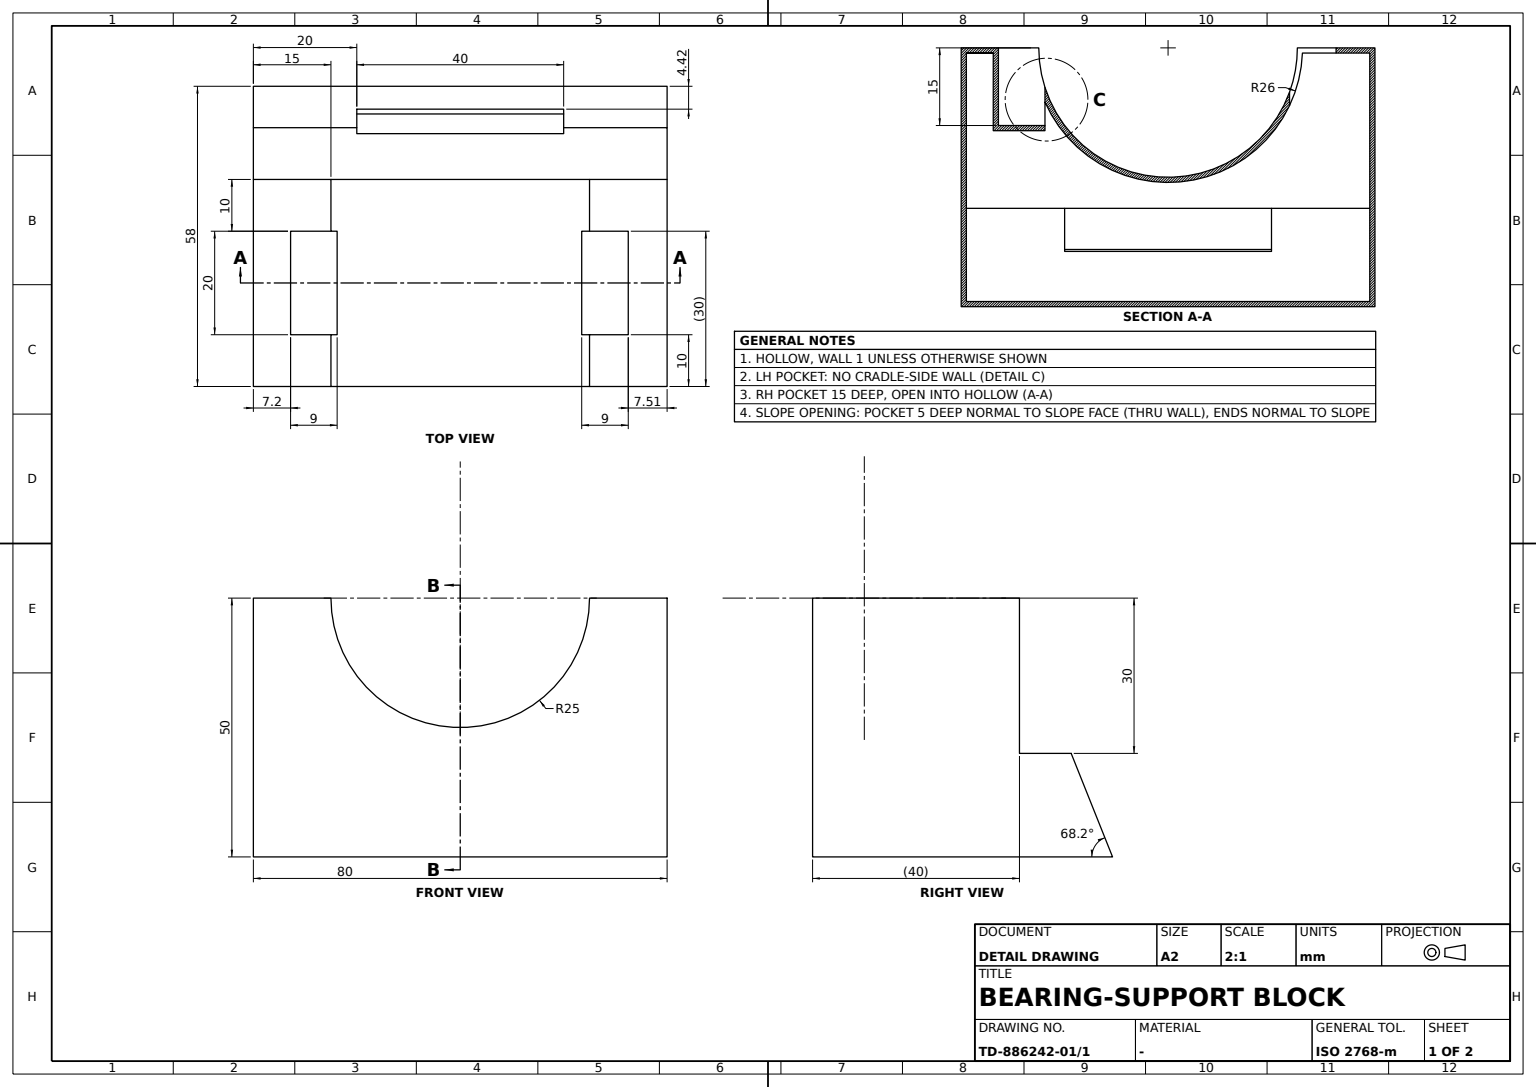
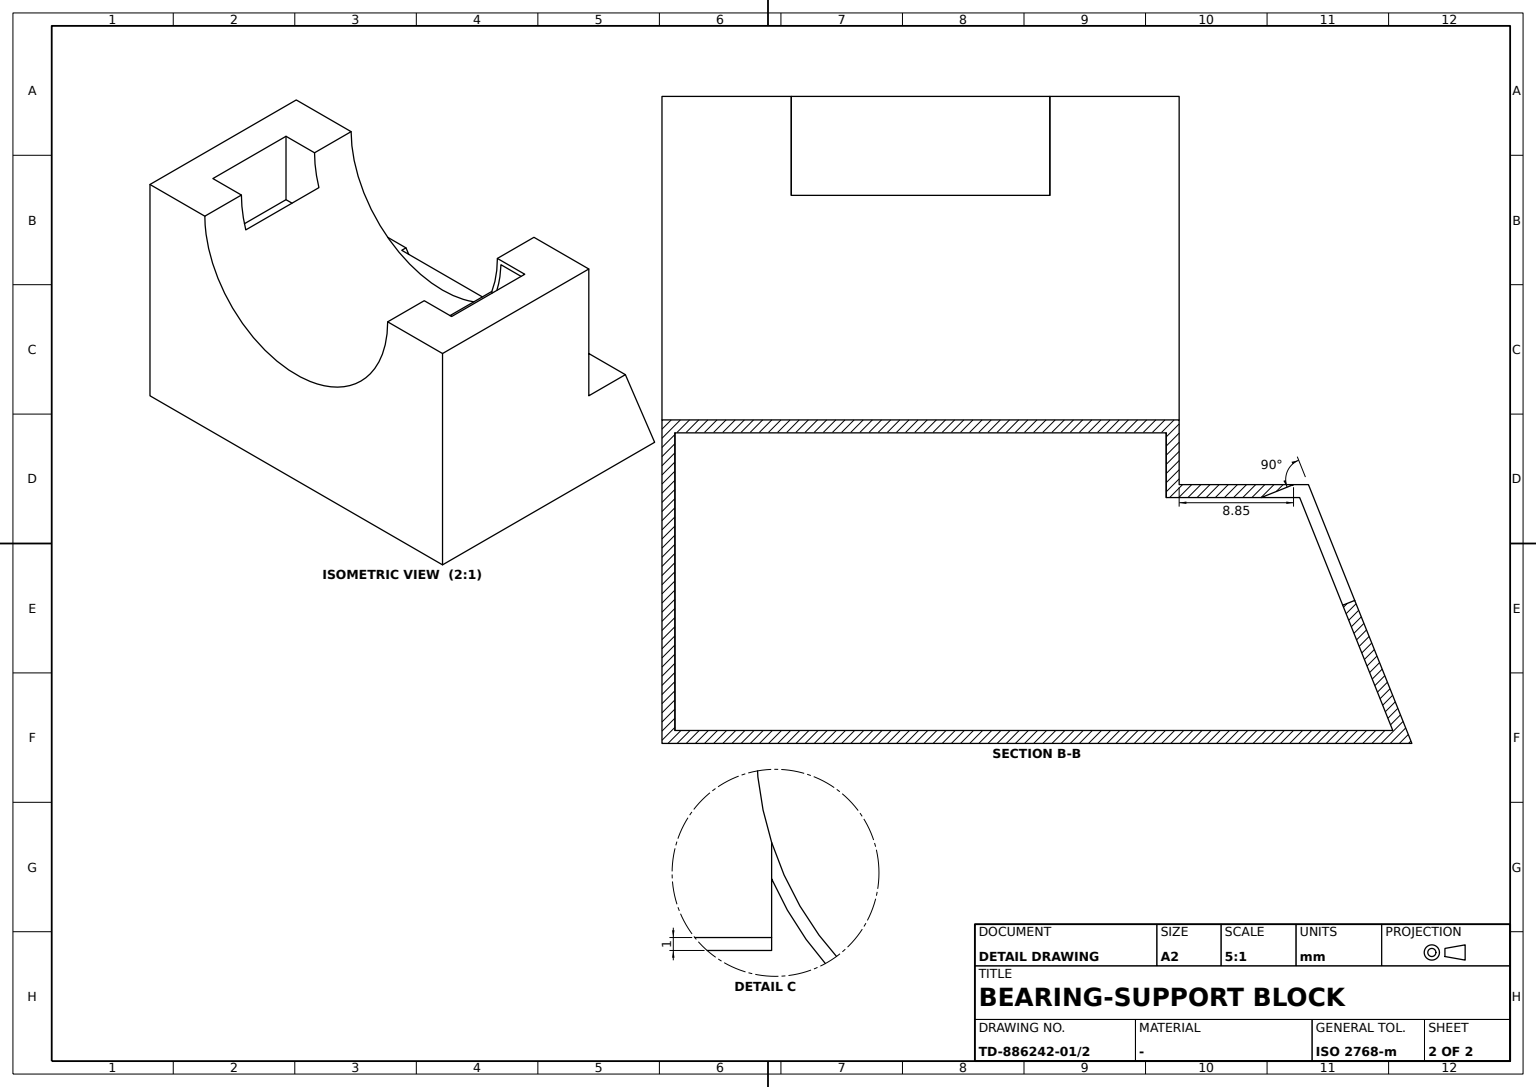
ISO-10303-21;
HEADER;
FILE_DESCRIPTION((''),'2;1');
FILE_NAME('','',(''),(''),'','','');
FILE_SCHEMA(('AUTOMOTIVE_DESIGN'));
ENDSEC;
DATA;
#1=APPLICATION_CONTEXT('');
#2=PRODUCT_CONTEXT('',#1,'mechanical');
#3=PRODUCT('','','',(#2));
#4=PRODUCT_DEFINITION_FORMATION('','',#3);
#5=PRODUCT_DEFINITION_CONTEXT('',#1,'design');
#6=PRODUCT_DEFINITION('','',#4,#5);
#7=PRODUCT_DEFINITION_SHAPE('','',#6);
#8=(LENGTH_UNIT()NAMED_UNIT(*)SI_UNIT(.MILLI.,.METRE.));
#9=(NAMED_UNIT(*)PLANE_ANGLE_UNIT()SI_UNIT($,.RADIAN.));
#10=(NAMED_UNIT(*)SI_UNIT($,.STERADIAN.)SOLID_ANGLE_UNIT());
#11=UNCERTAINTY_MEASURE_WITH_UNIT(LENGTH_MEASURE(0.005),#8,'distance_accuracy_value','');
#12=(GEOMETRIC_REPRESENTATION_CONTEXT(3)GLOBAL_UNCERTAINTY_ASSIGNED_CONTEXT((#11))GLOBAL_UNIT_ASSIGNED_CONTEXT((#8,#9,#10))REPRESENTATION_CONTEXT('',''));
#13=CARTESIAN_POINT('',(-80.,11.,25.));
#14=VERTEX_POINT('',#13);
#15=CARTESIAN_POINT('',(-80.,-29.,25.));
#16=VERTEX_POINT('',#15);
#17=DIRECTION('',(0.,-1.,0.));
#18=VECTOR('',#17,1000.);
#19=LINE('',#13,#18);
#20=EDGE_CURVE('',#14,#16,#19,.T.);
#21=ORIENTED_EDGE('',*,*,#20,.F.);
#22=CARTESIAN_POINT('',(-80.,11.,-5.));
#23=VERTEX_POINT('',#22);
#24=DIRECTION('',(0.,0.,1.));
#25=VECTOR('',#24,1000.);
#26=LINE('',#22,#25);
#27=EDGE_CURVE('',#23,#14,#26,.T.);
#28=ORIENTED_EDGE('',*,*,#27,.F.);
#29=CARTESIAN_POINT('',(-80.,21.,-5.));
#30=VERTEX_POINT('',#29);
#31=LINE('',#29,#18);
#32=EDGE_CURVE('',#30,#23,#31,.T.);
#33=ORIENTED_EDGE('',*,*,#32,.F.);
#34=CARTESIAN_POINT('',(-80.,29.,-25.));
#35=VERTEX_POINT('',#34);
#36=DIRECTION('',(0.,-0.371390676,0.928476691));
#37=VECTOR('',#36,1000.);
#38=LINE('',#34,#37);
#39=EDGE_CURVE('',#35,#30,#38,.T.);
#40=ORIENTED_EDGE('',*,*,#39,.F.);
#41=CARTESIAN_POINT('',(-80.,-29.,-25.));
#42=VERTEX_POINT('',#41);
#43=DIRECTION('',(0.,1.,0.));
#44=VECTOR('',#43,1000.);
#45=LINE('',#41,#44);
#46=EDGE_CURVE('',#42,#35,#45,.T.);
#47=ORIENTED_EDGE('',*,*,#46,.F.);
#48=DIRECTION('',(0.,0.,-1.));
#49=VECTOR('',#48,1000.);
#50=LINE('',#15,#49);
#51=EDGE_CURVE('',#16,#42,#50,.T.);
#52=ORIENTED_EDGE('',*,*,#51,.F.);
#53=EDGE_LOOP('',(#21,#28,#33,#40,#47,#52));
#54=FACE_BOUND('',#53,.T.);
#55=CARTESIAN_POINT('',(-80.,0.,0.));
#56=DIRECTION('',(1.,0.,0.));
#57=AXIS2_PLACEMENT_3D('',#55,#56,#43);
#58=PLANE('',#57);
#59=ADVANCED_FACE('',(#54),#58,.F.);
#60=CARTESIAN_POINT('',(-63.80175,2.,9.));
#61=VERTEX_POINT('',#60);
#62=CARTESIAN_POINT('',(-63.80175,-20.,9.));
#63=VERTEX_POINT('',#62);
#64=CARTESIAN_POINT('',(-63.80175,0.,9.));
#65=LINE('',#64,#18);
#66=EDGE_CURVE('',#61,#63,#65,.T.);
#67=ORIENTED_EDGE('',*,*,#66,.F.);
#68=CARTESIAN_POINT('',(-63.80175,2.,14.536889));
#69=VERTEX_POINT('',#68);
#70=CARTESIAN_POINT('',(-63.80175,2.,25.));
#71=LINE('',#70,#49);
#72=EDGE_CURVE('',#69,#61,#71,.T.);
#73=ORIENTED_EDGE('',*,*,#72,.F.);
#74=CARTESIAN_POINT('',(-63.80175,1.,14.536889));
#75=VERTEX_POINT('',#74);
#76=LINE('',#68,#44);
#77=EDGE_CURVE('',#69,#75,#76,.F.);
#78=ORIENTED_EDGE('',*,*,#77,.T.);
#79=CARTESIAN_POINT('',(-63.80175,1.,10.));
#80=VERTEX_POINT('',#79);
#81=CARTESIAN_POINT('',(-63.80175,1.,25.));
#82=LINE('',#81,#49);
#83=EDGE_CURVE('',#75,#80,#82,.T.);
#84=ORIENTED_EDGE('',*,*,#83,.T.);
#85=CARTESIAN_POINT('',(-63.80175,-19.,10.));
#86=VERTEX_POINT('',#85);
#87=LINE('',#85,#44);
#88=EDGE_CURVE('',#86,#80,#87,.T.);
#89=ORIENTED_EDGE('',*,*,#88,.F.);
#90=CARTESIAN_POINT('',(-63.80175,-19.,14.536889));
#91=VERTEX_POINT('',#90);
#92=CARTESIAN_POINT('',(-63.80175,-19.,25.));
#93=LINE('',#92,#49);
#94=EDGE_CURVE('',#91,#86,#93,.T.);
#95=ORIENTED_EDGE('',*,*,#94,.F.);
#96=CARTESIAN_POINT('',(-63.80175,-20.,14.536889));
#97=VERTEX_POINT('',#96);
#98=LINE('',#90,#44);
#99=EDGE_CURVE('',#91,#97,#98,.F.);
#100=ORIENTED_EDGE('',*,*,#99,.T.);
#101=CARTESIAN_POINT('',(-63.80175,-20.,25.));
#102=LINE('',#101,#49);
#103=EDGE_CURVE('',#97,#63,#102,.T.);
#104=ORIENTED_EDGE('',*,*,#103,.T.);
#105=EDGE_LOOP('',(#67,#73,#78,#84,#89,#95,#100,#104));
#106=FACE_BOUND('',#105,.T.);
#107=DIRECTION('',(-1.,0.,0.));
#108=AXIS2_PLACEMENT_3D('',#92,#107,#43);
#109=PLANE('',#108);
#110=ADVANCED_FACE('',(#106),#109,.F.);
#111=CARTESIAN_POINT('',(-16.511753,-19.,16.438326));
#112=VERTEX_POINT('',#111);
#113=CARTESIAN_POINT('',(-16.511753,-19.,13.850908));
#114=VERTEX_POINT('',#113);
#115=CARTESIAN_POINT('',(-16.511753,-19.,25.));
#116=LINE('',#115,#49);
#117=EDGE_CURVE('',#112,#114,#116,.T.);
#118=ORIENTED_EDGE('',*,*,#117,.F.);
#119=CARTESIAN_POINT('',(-15.,-19.,25.));
#120=VERTEX_POINT('',#119);
#121=CARTESIAN_POINT('',(-40.,-19.,25.));
#122=AXIS2_PLACEMENT_3D('',#121,#17,#48);
#123=CIRCLE('',#122,25.);
#124=EDGE_CURVE('',#112,#120,#123,.T.);
#125=ORIENTED_EDGE('',*,*,#124,.T.);
#126=CARTESIAN_POINT('',(-7.511753,-19.,25.));
#127=VERTEX_POINT('',#126);
#128=CARTESIAN_POINT('',(0.,-19.,25.));
#129=VECTOR('',#107,1000.);
#130=LINE('',#128,#129);
#131=EDGE_CURVE('',#127,#120,#130,.T.);
#132=ORIENTED_EDGE('',*,*,#131,.F.);
#133=CARTESIAN_POINT('',(-7.511753,-19.,24.));
#134=VERTEX_POINT('',#133);
#135=LINE('',#126,#49);
#136=EDGE_CURVE('',#127,#134,#135,.T.);
#137=ORIENTED_EDGE('',*,*,#136,.T.);
#138=CARTESIAN_POINT('',(-14.019238,-19.,24.));
#139=VERTEX_POINT('',#138);
#140=CARTESIAN_POINT('',(-63.80175,-19.,24.));
#141=VECTOR('',#56,1000.);
#142=LINE('',#140,#141);
#143=EDGE_CURVE('',#139,#134,#142,.T.);
#144=ORIENTED_EDGE('',*,*,#143,.F.);
#145=CIRCLE('',#122,26.);
#146=EDGE_CURVE('',#114,#139,#145,.T.);
#147=ORIENTED_EDGE('',*,*,#146,.F.);
#148=EDGE_LOOP('',(#118,#125,#132,#137,#144,#147));
#149=FACE_BOUND('',#148,.T.);
#150=AXIS2_PLACEMENT_3D('',#92,#17,#107);
#151=PLANE('',#150);
#152=ADVANCED_FACE('',(#149),#151,.F.);
#153=ORIENTED_EDGE('',*,*,#27,.T.);
#154=CARTESIAN_POINT('',(-65.,11.,25.));
#155=VERTEX_POINT('',#154);
#156=CARTESIAN_POINT('',(0.,11.,25.));
#157=LINE('',#156,#129);
#158=EDGE_CURVE('',#155,#14,#157,.T.);
#159=ORIENTED_EDGE('',*,*,#158,.F.);
#160=CARTESIAN_POINT('',(-15.,11.,25.));
#161=VERTEX_POINT('',#160);
#162=CARTESIAN_POINT('',(-40.,11.,25.));
#163=AXIS2_PLACEMENT_3D('',#162,#17,#48);
#164=CIRCLE('',#163,25.);
#165=EDGE_CURVE('',#161,#155,#164,.F.);
#166=ORIENTED_EDGE('',*,*,#165,.F.);
#167=VERTEX_POINT('',#156);
#168=EDGE_CURVE('',#167,#161,#157,.T.);
#169=ORIENTED_EDGE('',*,*,#168,.F.);
#170=CARTESIAN_POINT('',(0.,11.,-5.));
#171=VERTEX_POINT('',#170);
#172=LINE('',#170,#25);
#173=EDGE_CURVE('',#171,#167,#172,.T.);
#174=ORIENTED_EDGE('',*,*,#173,.F.);
#175=LINE('',#170,#129);
#176=EDGE_CURVE('',#171,#23,#175,.T.);
#177=ORIENTED_EDGE('',*,*,#176,.T.);
#178=EDGE_LOOP('',(#153,#159,#166,#169,#174,#177));
#179=FACE_BOUND('',#178,.T.);
#180=AXIS2_PLACEMENT_3D('',#170,#17,#24);
#181=PLANE('',#180);
#182=ADVANCED_FACE('',(#179),#181,.F.);
#183=CARTESIAN_POINT('',(0.,29.,-25.));
#184=VERTEX_POINT('',#183);
#185=CARTESIAN_POINT('',(0.,21.,-5.));
#186=VERTEX_POINT('',#185);
#187=LINE('',#183,#37);
#188=EDGE_CURVE('',#184,#186,#187,.T.);
#189=ORIENTED_EDGE('',*,*,#188,.T.);
#190=LINE('',#185,#18);
#191=EDGE_CURVE('',#186,#171,#190,.T.);
#192=ORIENTED_EDGE('',*,*,#191,.T.);
#193=ORIENTED_EDGE('',*,*,#173,.T.);
#194=CARTESIAN_POINT('',(0.,-29.,25.));
#195=VERTEX_POINT('',#194);
#196=LINE('',#156,#18);
#197=EDGE_CURVE('',#167,#195,#196,.T.);
#198=ORIENTED_EDGE('',*,*,#197,.T.);
#199=CARTESIAN_POINT('',(0.,-29.,-25.));
#200=VERTEX_POINT('',#199);
#201=LINE('',#194,#49);
#202=EDGE_CURVE('',#195,#200,#201,.T.);
#203=ORIENTED_EDGE('',*,*,#202,.T.);
#204=LINE('',#199,#44);
#205=EDGE_CURVE('',#200,#184,#204,.T.);
#206=ORIENTED_EDGE('',*,*,#205,.T.);
#207=EDGE_LOOP('',(#189,#192,#193,#198,#203,#206));
#208=FACE_BOUND('',#207,.T.);
#209=CARTESIAN_POINT('',(0.,0.,0.));
#210=AXIS2_PLACEMENT_3D('',#209,#56,#43);
#211=PLANE('',#210);
#212=ADVANCED_FACE('',(#208),#211,.T.);
#213=CARTESIAN_POINT('',(-63.80175,1.,17.352995));
#214=VERTEX_POINT('',#213);
#215=CARTESIAN_POINT('',(-65.,1.,25.));
#216=VERTEX_POINT('',#215);
#217=CARTESIAN_POINT('',(-40.,1.,25.));
#218=AXIS2_PLACEMENT_3D('',#217,#43,#24);
#219=CIRCLE('',#218,25.);
#220=EDGE_CURVE('',#214,#216,#219,.T.);
#221=ORIENTED_EDGE('',*,*,#220,.T.);
#222=CARTESIAN_POINT('',(-72.80175,1.,25.));
#223=VERTEX_POINT('',#222);
#224=CARTESIAN_POINT('',(0.,1.,25.));
#225=LINE('',#224,#141);
#226=EDGE_CURVE('',#223,#216,#225,.T.);
#227=ORIENTED_EDGE('',*,*,#226,.F.);
#228=CARTESIAN_POINT('',(-72.80175,1.,10.));
#229=VERTEX_POINT('',#228);
#230=LINE('',#222,#49);
#231=EDGE_CURVE('',#223,#229,#230,.T.);
#232=ORIENTED_EDGE('',*,*,#231,.T.);
#233=LINE('',#228,#141);
#234=EDGE_CURVE('',#229,#80,#233,.T.);
#235=ORIENTED_EDGE('',*,*,#234,.T.);
#236=ORIENTED_EDGE('',*,*,#83,.F.);
#237=EDGE_CURVE('',#214,#75,#82,.T.);
#238=ORIENTED_EDGE('',*,*,#237,.F.);
#239=EDGE_LOOP('',(#221,#227,#232,#235,#236,#238));
#240=FACE_BOUND('',#239,.T.);
#241=AXIS2_PLACEMENT_3D('',#222,#43,#56);
#242=PLANE('',#241);
#243=ADVANCED_FACE('',(#240),#242,.F.);
#244=CARTESIAN_POINT('',(-73.80175,2.,9.));
#245=VERTEX_POINT('',#244);
#246=CARTESIAN_POINT('',(-72.80175,2.,9.));
#247=LINE('',#246,#141);
#248=EDGE_CURVE('',#245,#61,#247,.T.);
#249=ORIENTED_EDGE('',*,*,#248,.T.);
#250=ORIENTED_EDGE('',*,*,#66,.T.);
#251=CARTESIAN_POINT('',(-73.80175,-20.,9.));
#252=VERTEX_POINT('',#251);
#253=CARTESIAN_POINT('',(0.,-20.,9.));
#254=LINE('',#253,#141);
#255=EDGE_CURVE('',#252,#63,#254,.T.);
#256=ORIENTED_EDGE('',*,*,#255,.F.);
#257=CARTESIAN_POINT('',(-73.80175,1.,9.));
#258=LINE('',#257,#18);
#259=EDGE_CURVE('',#245,#252,#258,.T.);
#260=ORIENTED_EDGE('',*,*,#259,.F.);
#261=EDGE_LOOP('',(#249,#250,#256,#260));
#262=FACE_BOUND('',#261,.T.);
#263=CARTESIAN_POINT('',(0.,0.,9.));
#264=AXIS2_PLACEMENT_3D('',#263,#24,#56);
#265=PLANE('',#264);
#266=ADVANCED_FACE('',(#262),#265,.F.);
#267=CARTESIAN_POINT('',(-65.980762,10.,24.));
#268=VERTEX_POINT('',#267);
#269=CARTESIAN_POINT('',(-14.019238,10.,24.));
#270=VERTEX_POINT('',#269);
#271=CARTESIAN_POINT('',(-40.,10.,25.));
#272=AXIS2_PLACEMENT_3D('',#271,#17,#48);
#273=CIRCLE('',#272,26.);
#274=EDGE_CURVE('',#268,#270,#273,.T.);
#275=ORIENTED_EDGE('',*,*,#274,.F.);
#276=CARTESIAN_POINT('',(-79.,10.,24.));
#277=VERTEX_POINT('',#276);
#278=CARTESIAN_POINT('',(0.,10.,24.));
#279=LINE('',#278,#141);
#280=EDGE_CURVE('',#277,#268,#279,.T.);
#281=ORIENTED_EDGE('',*,*,#280,.F.);
#282=CARTESIAN_POINT('',(-79.,10.,-6.));
#283=VERTEX_POINT('',#282);
#284=CARTESIAN_POINT('',(-79.,10.,0.));
#285=LINE('',#284,#49);
#286=EDGE_CURVE('',#277,#283,#285,.T.);
#287=ORIENTED_EDGE('',*,*,#286,.T.);
#288=CARTESIAN_POINT('',(-1.,10.,-6.));
#289=VERTEX_POINT('',#288);
#290=CARTESIAN_POINT('',(0.,10.,-6.));
#291=LINE('',#290,#141);
#292=EDGE_CURVE('',#283,#289,#291,.T.);
#293=ORIENTED_EDGE('',*,*,#292,.T.);
#294=CARTESIAN_POINT('',(-1.,10.,24.));
#295=VERTEX_POINT('',#294);
#296=CARTESIAN_POINT('',(-1.,10.,-5.));
#297=LINE('',#296,#25);
#298=EDGE_CURVE('',#289,#295,#297,.T.);
#299=ORIENTED_EDGE('',*,*,#298,.T.);
#300=EDGE_CURVE('',#270,#295,#279,.T.);
#301=ORIENTED_EDGE('',*,*,#300,.F.);
#302=EDGE_LOOP('',(#275,#281,#287,#293,#299,#301));
#303=FACE_BOUND('',#302,.T.);
#304=CARTESIAN_POINT('',(0.,10.,-5.));
#305=AXIS2_PLACEMENT_3D('',#304,#17,#24);
#306=PLANE('',#305);
#307=ADVANCED_FACE('',(#303),#306,.T.);
#308=CARTESIAN_POINT('',(-79.,-28.,24.));
#309=VERTEX_POINT('',#308);
#310=CARTESIAN_POINT('',(-79.,-28.,-24.));
#311=VERTEX_POINT('',#310);
#312=CARTESIAN_POINT('',(-79.,-28.,25.));
#313=LINE('',#312,#49);
#314=EDGE_CURVE('',#309,#311,#313,.T.);
#315=ORIENTED_EDGE('',*,*,#314,.F.);
#316=CARTESIAN_POINT('',(-65.980762,-28.,24.));
#317=VERTEX_POINT('',#316);
#318=CARTESIAN_POINT('',(0.,-28.,24.));
#319=LINE('',#318,#129);
#320=EDGE_CURVE('',#317,#309,#319,.T.);
#321=ORIENTED_EDGE('',*,*,#320,.F.);
#322=CARTESIAN_POINT('',(-14.019238,-28.,24.));
#323=VERTEX_POINT('',#322);
#324=CARTESIAN_POINT('',(-40.,-28.,25.));
#325=AXIS2_PLACEMENT_3D('',#324,#43,#24);
#326=CIRCLE('',#325,26.);
#327=EDGE_CURVE('',#323,#317,#326,.T.);
#328=ORIENTED_EDGE('',*,*,#327,.F.);
#329=CARTESIAN_POINT('',(-1.,-28.,24.));
#330=VERTEX_POINT('',#329);
#331=EDGE_CURVE('',#330,#323,#319,.T.);
#332=ORIENTED_EDGE('',*,*,#331,.F.);
#333=CARTESIAN_POINT('',(-1.,-28.,-24.));
#334=VERTEX_POINT('',#333);
#335=CARTESIAN_POINT('',(-1.,-28.,0.));
#336=LINE('',#335,#25);
#337=EDGE_CURVE('',#334,#330,#336,.T.);
#338=ORIENTED_EDGE('',*,*,#337,.F.);
#339=CARTESIAN_POINT('',(0.,-28.,-24.));
#340=LINE('',#339,#141);
#341=EDGE_CURVE('',#311,#334,#340,.T.);
#342=ORIENTED_EDGE('',*,*,#341,.F.);
#343=EDGE_LOOP('',(#315,#321,#328,#332,#338,#342));
#344=FACE_BOUND('',#343,.T.);
#345=CARTESIAN_POINT('',(0.,-28.,25.));
#346=AXIS2_PLACEMENT_3D('',#345,#43,#48);
#347=PLANE('',#346);
#348=ADVANCED_FACE('',(#344),#347,.T.);
#349=LINE('',#154,#44);
#350=EDGE_CURVE('',#216,#155,#349,.T.);
#351=ORIENTED_EDGE('',*,*,#350,.F.);
#352=ORIENTED_EDGE('',*,*,#220,.F.);
#353=CARTESIAN_POINT('',(-63.80175,-19.,17.352995));
#354=VERTEX_POINT('',#353);
#355=LINE('',#353,#44);
#356=EDGE_CURVE('',#354,#214,#355,.T.);
#357=ORIENTED_EDGE('',*,*,#356,.F.);
#358=CARTESIAN_POINT('',(-65.,-19.,25.));
#359=VERTEX_POINT('',#358);
#360=EDGE_CURVE('',#359,#354,#123,.T.);
#361=ORIENTED_EDGE('',*,*,#360,.F.);
#362=CARTESIAN_POINT('',(-65.,-29.,25.));
#363=VERTEX_POINT('',#362);
#364=LINE('',#358,#44);
#365=EDGE_CURVE('',#363,#359,#364,.T.);
#366=ORIENTED_EDGE('',*,*,#365,.F.);
#367=CARTESIAN_POINT('',(-15.,-29.,25.));
#368=VERTEX_POINT('',#367);
#369=CARTESIAN_POINT('',(-40.,-29.,25.));
#370=AXIS2_PLACEMENT_3D('',#369,#43,#24);
#371=CIRCLE('',#370,25.);
#372=EDGE_CURVE('',#368,#363,#371,.T.);
#373=ORIENTED_EDGE('',*,*,#372,.F.);
#374=LINE('',#119,#44);
#375=EDGE_CURVE('',#120,#368,#374,.F.);
#376=ORIENTED_EDGE('',*,*,#375,.F.);
#377=ORIENTED_EDGE('',*,*,#124,.F.);
#378=CARTESIAN_POINT('',(-16.511753,1.,16.438326));
#379=VERTEX_POINT('',#378);
#380=LINE('',#378,#44);
#381=EDGE_CURVE('',#379,#112,#380,.F.);
#382=ORIENTED_EDGE('',*,*,#381,.F.);
#383=CARTESIAN_POINT('',(-15.,1.,25.));
#384=VERTEX_POINT('',#383);
#385=EDGE_CURVE('',#384,#379,#219,.T.);
#386=ORIENTED_EDGE('',*,*,#385,.F.);
#387=LINE('',#160,#44);
#388=EDGE_CURVE('',#161,#384,#387,.F.);
#389=ORIENTED_EDGE('',*,*,#388,.F.);
#390=ORIENTED_EDGE('',*,*,#165,.T.);
#391=EDGE_LOOP('',(#351,#352,#357,#361,#366,#373,#376,#377,#382,#386,#389,#390));
#392=FACE_BOUND('',#391,.T.);
#393=CARTESIAN_POINT('',(-40.,-9.66,25.));
#394=AXIS2_PLACEMENT_3D('',#393,#43,#107);
#395=CYLINDRICAL_SURFACE('',#394,25.);
#396=ADVANCED_FACE('',(#392),#395,.F.);
#397=ORIENTED_EDGE('',*,*,#51,.T.);
#398=LINE('',#199,#129);
#399=EDGE_CURVE('',#200,#42,#398,.T.);
#400=ORIENTED_EDGE('',*,*,#399,.F.);
#401=ORIENTED_EDGE('',*,*,#202,.F.);
#402=LINE('',#194,#129);
#403=EDGE_CURVE('',#195,#368,#402,.T.);
#404=ORIENTED_EDGE('',*,*,#403,.T.);
#405=ORIENTED_EDGE('',*,*,#372,.T.);
#406=EDGE_CURVE('',#363,#16,#402,.T.);
#407=ORIENTED_EDGE('',*,*,#406,.T.);
#408=EDGE_LOOP('',(#397,#400,#401,#404,#405,#407));
#409=FACE_BOUND('',#408,.T.);
#410=AXIS2_PLACEMENT_3D('',#194,#43,#48);
#411=PLANE('',#410);
#412=ADVANCED_FACE('',(#409),#411,.F.);
#413=CARTESIAN_POINT('',(-20.,17.347057,-6.));
#414=VERTEX_POINT('',#413);
#415=CARTESIAN_POINT('',(-60.,17.347057,-6.));
#416=VERTEX_POINT('',#415);
#417=CARTESIAN_POINT('',(0.,17.347057,-6.));
#418=LINE('',#417,#129);
#419=EDGE_CURVE('',#414,#416,#418,.T.);
#420=ORIENTED_EDGE('',*,*,#419,.T.);
#421=CARTESIAN_POINT('',(-60.,19.847057,-5.));
#422=VERTEX_POINT('',#421);
#423=CARTESIAN_POINT('',(-60.,20.840973,-4.602434));
#424=DIRECTION('',(0.,-0.928476691,-0.371390676));
#425=VECTOR('',#424,1000.);
#426=LINE('',#423,#425);
#427=EDGE_CURVE('',#422,#416,#426,.T.);
#428=ORIENTED_EDGE('',*,*,#427,.F.);
#429=CARTESIAN_POINT('',(-20.,19.847057,-5.));
#430=VERTEX_POINT('',#429);
#431=CARTESIAN_POINT('',(0.,19.847057,-5.));
#432=LINE('',#431,#129);
#433=EDGE_CURVE('',#430,#422,#432,.T.);
#434=ORIENTED_EDGE('',*,*,#433,.F.);
#435=CARTESIAN_POINT('',(-20.,20.840973,-4.602434));
#436=LINE('',#435,#425);
#437=EDGE_CURVE('',#430,#414,#436,.T.);
#438=ORIENTED_EDGE('',*,*,#437,.T.);
#439=EDGE_LOOP('',(#420,#428,#434,#438));
#440=FACE_BOUND('',#439,.T.);
#441=AXIS2_PLACEMENT_3D('',#435,#36,#107);
#442=PLANE('',#441);
#443=ADVANCED_FACE('',(#440),#442,.F.);
#444=CARTESIAN_POINT('',(-1.,11.,24.));
#445=LINE('',#444,#18);
#446=EDGE_CURVE('',#295,#330,#445,.T.);
#447=ORIENTED_EDGE('',*,*,#446,.F.);
#448=ORIENTED_EDGE('',*,*,#298,.F.);
#449=CARTESIAN_POINT('',(-1.,20.322967,-6.));
#450=VERTEX_POINT('',#449);
#451=CARTESIAN_POINT('',(-1.,0.,-6.));
#452=LINE('',#451,#44);
#453=EDGE_CURVE('',#289,#450,#452,.T.);
#454=ORIENTED_EDGE('',*,*,#453,.T.);
#455=CARTESIAN_POINT('',(-1.,27.522967,-24.));
#456=VERTEX_POINT('',#455);
#457=CARTESIAN_POINT('',(-1.,15.450834,6.180333));
#458=DIRECTION('',(0.,0.371390676,-0.928476691));
#459=VECTOR('',#458,1000.);
#460=LINE('',#457,#459);
#461=EDGE_CURVE('',#450,#456,#460,.T.);
#462=ORIENTED_EDGE('',*,*,#461,.T.);
#463=CARTESIAN_POINT('',(-1.,0.,-24.));
#464=LINE('',#463,#18);
#465=EDGE_CURVE('',#456,#334,#464,.T.);
#466=ORIENTED_EDGE('',*,*,#465,.T.);
#467=ORIENTED_EDGE('',*,*,#337,.T.);
#468=EDGE_LOOP('',(#447,#448,#454,#462,#466,#467));
#469=FACE_BOUND('',#468,.T.);
#470=CARTESIAN_POINT('',(-1.,0.,0.));
#471=AXIS2_PLACEMENT_3D('',#470,#56,#43);
#472=PLANE('',#471);
#473=ADVANCED_FACE('',(#469),#472,.F.);
#474=CARTESIAN_POINT('',(-65.980762,2.,24.));
#475=VERTEX_POINT('',#474);
#476=CARTESIAN_POINT('',(-40.,2.,25.));
#477=AXIS2_PLACEMENT_3D('',#476,#43,#24);
#478=CIRCLE('',#477,26.);
#479=EDGE_CURVE('',#475,#69,#478,.F.);
#480=ORIENTED_EDGE('',*,*,#479,.T.);
#481=ORIENTED_EDGE('',*,*,#72,.T.);
#482=ORIENTED_EDGE('',*,*,#248,.F.);
#483=CARTESIAN_POINT('',(-73.80175,2.,24.));
#484=VERTEX_POINT('',#483);
#485=CARTESIAN_POINT('',(-73.80175,2.,25.));
#486=LINE('',#485,#49);
#487=EDGE_CURVE('',#484,#245,#486,.T.);
#488=ORIENTED_EDGE('',*,*,#487,.F.);
#489=CARTESIAN_POINT('',(-72.80175,2.,24.));
#490=LINE('',#489,#129);
#491=EDGE_CURVE('',#475,#484,#490,.T.);
#492=ORIENTED_EDGE('',*,*,#491,.F.);
#493=EDGE_LOOP('',(#480,#481,#482,#488,#492));
#494=FACE_BOUND('',#493,.T.);
#495=CARTESIAN_POINT('',(-72.80175,2.,25.));
#496=AXIS2_PLACEMENT_3D('',#495,#43,#56);
#497=PLANE('',#496);
#498=ADVANCED_FACE('',(#494),#497,.T.);
#499=ORIENTED_EDGE('',*,*,#205,.F.);
#500=ORIENTED_EDGE('',*,*,#399,.T.);
#501=ORIENTED_EDGE('',*,*,#46,.T.);
#502=LINE('',#183,#129);
#503=EDGE_CURVE('',#184,#35,#502,.T.);
#504=ORIENTED_EDGE('',*,*,#503,.F.);
#505=EDGE_LOOP('',(#499,#500,#501,#504));
#506=FACE_BOUND('',#505,.T.);
#507=AXIS2_PLACEMENT_3D('',#199,#24,#43);
#508=PLANE('',#507);
#509=ADVANCED_FACE('',(#506),#508,.F.);
#510=ORIENTED_EDGE('',*,*,#237,.T.);
#511=LINE('',#74,#44);
#512=EDGE_CURVE('',#75,#91,#511,.F.);
#513=ORIENTED_EDGE('',*,*,#512,.T.);
#514=EDGE_CURVE('',#354,#91,#93,.T.);
#515=ORIENTED_EDGE('',*,*,#514,.F.);
#516=ORIENTED_EDGE('',*,*,#356,.T.);
#517=EDGE_LOOP('',(#510,#513,#515,#516));
#518=FACE_BOUND('',#517,.T.);
#519=ADVANCED_FACE('',(#518),#109,.T.);
#520=CARTESIAN_POINT('',(-60.,21.,-5.));
#521=VERTEX_POINT('',#520);
#522=LINE('',#185,#129);
#523=EDGE_CURVE('',#521,#30,#522,.T.);
#524=ORIENTED_EDGE('',*,*,#523,.T.);
#525=ORIENTED_EDGE('',*,*,#32,.T.);
#526=ORIENTED_EDGE('',*,*,#176,.F.);
#527=ORIENTED_EDGE('',*,*,#191,.F.);
#528=CARTESIAN_POINT('',(-20.,21.,-5.));
#529=VERTEX_POINT('',#528);
#530=EDGE_CURVE('',#186,#529,#522,.T.);
#531=ORIENTED_EDGE('',*,*,#530,.T.);
#532=CARTESIAN_POINT('',(-20.,20.840973,-5.));
#533=LINE('',#532,#18);
#534=EDGE_CURVE('',#529,#430,#533,.T.);
#535=ORIENTED_EDGE('',*,*,#534,.T.);
#536=ORIENTED_EDGE('',*,*,#433,.T.);
#537=LINE('',#520,#18);
#538=EDGE_CURVE('',#521,#422,#537,.T.);
#539=ORIENTED_EDGE('',*,*,#538,.F.);
#540=EDGE_LOOP('',(#524,#525,#526,#527,#531,#535,#536,#539));
#541=FACE_BOUND('',#540,.T.);
#542=AXIS2_PLACEMENT_3D('',#185,#48,#17);
#543=PLANE('',#542);
#544=ADVANCED_FACE('',(#541),#543,.F.);
#545=ORIENTED_EDGE('',*,*,#465,.F.);
#546=CARTESIAN_POINT('',(-79.,27.522967,-24.));
#547=VERTEX_POINT('',#546);
#548=CARTESIAN_POINT('',(0.,27.522967,-24.));
#549=LINE('',#548,#141);
#550=EDGE_CURVE('',#547,#456,#549,.T.);
#551=ORIENTED_EDGE('',*,*,#550,.F.);
#552=CARTESIAN_POINT('',(-79.,-29.,-24.));
#553=LINE('',#552,#44);
#554=EDGE_CURVE('',#311,#547,#553,.T.);
#555=ORIENTED_EDGE('',*,*,#554,.F.);
#556=ORIENTED_EDGE('',*,*,#341,.T.);
#557=EDGE_LOOP('',(#545,#551,#555,#556));
#558=FACE_BOUND('',#557,.T.);
#559=CARTESIAN_POINT('',(0.,-29.,-24.));
#560=AXIS2_PLACEMENT_3D('',#559,#24,#43);
#561=PLANE('',#560);
#562=ADVANCED_FACE('',(#558),#561,.T.);
#563=CARTESIAN_POINT('',(-65.980762,-20.,24.));
#564=VERTEX_POINT('',#563);
#565=LINE('',#316,#44);
#566=EDGE_CURVE('',#317,#564,#565,.T.);
#567=ORIENTED_EDGE('',*,*,#566,.T.);
#568=CARTESIAN_POINT('',(-40.,-20.,25.));
#569=AXIS2_PLACEMENT_3D('',#568,#17,#48);
#570=CIRCLE('',#569,26.);
#571=EDGE_CURVE('',#564,#97,#570,.T.);
#572=ORIENTED_EDGE('',*,*,#571,.T.);
#573=ORIENTED_EDGE('',*,*,#99,.F.);
#574=ORIENTED_EDGE('',*,*,#512,.F.);
#575=ORIENTED_EDGE('',*,*,#77,.F.);
#576=ORIENTED_EDGE('',*,*,#479,.F.);
#577=LINE('',#474,#44);
#578=EDGE_CURVE('',#475,#268,#577,.T.);
#579=ORIENTED_EDGE('',*,*,#578,.T.);
#580=ORIENTED_EDGE('',*,*,#274,.T.);
#581=CARTESIAN_POINT('',(-14.019238,1.,24.));
#582=VERTEX_POINT('',#581);
#583=LINE('',#269,#44);
#584=EDGE_CURVE('',#270,#582,#583,.F.);
#585=ORIENTED_EDGE('',*,*,#584,.T.);
#586=CARTESIAN_POINT('',(-16.511753,1.,13.850908));
#587=VERTEX_POINT('',#586);
#588=CIRCLE('',#218,26.);
#589=EDGE_CURVE('',#582,#587,#588,.T.);
#590=ORIENTED_EDGE('',*,*,#589,.T.);
#591=LINE('',#586,#44);
#592=EDGE_CURVE('',#587,#114,#591,.F.);
#593=ORIENTED_EDGE('',*,*,#592,.T.);
#594=ORIENTED_EDGE('',*,*,#146,.T.);
#595=LINE('',#138,#44);
#596=EDGE_CURVE('',#139,#323,#595,.F.);
#597=ORIENTED_EDGE('',*,*,#596,.T.);
#598=ORIENTED_EDGE('',*,*,#327,.T.);
#599=EDGE_LOOP('',(#567,#572,#573,#574,#575,#576,#579,#580,#585,#590,#593,#594,#597,#598));
#600=FACE_BOUND('',#599,.T.);
#601=CYLINDRICAL_SURFACE('',#394,26.);
#602=ADVANCED_FACE('',(#600),#601,.T.);
#603=CARTESIAN_POINT('',(-16.511753,1.,25.));
#604=LINE('',#603,#49);
#605=EDGE_CURVE('',#379,#587,#604,.T.);
#606=ORIENTED_EDGE('',*,*,#605,.F.);
#607=ORIENTED_EDGE('',*,*,#381,.T.);
#608=ORIENTED_EDGE('',*,*,#117,.T.);
#609=ORIENTED_EDGE('',*,*,#592,.F.);
#610=EDGE_LOOP('',(#606,#607,#608,#609));
#611=FACE_BOUND('',#610,.T.);
#612=AXIS2_PLACEMENT_3D('',#603,#56,#17);
#613=PLANE('',#612);
#614=ADVANCED_FACE('',(#611),#613,.T.);
#615=CARTESIAN_POINT('',(-79.,20.322967,-6.));
#616=VERTEX_POINT('',#615);
#617=CARTESIAN_POINT('',(-79.,0.,-6.));
#618=LINE('',#617,#44);
#619=EDGE_CURVE('',#283,#616,#618,.T.);
#620=ORIENTED_EDGE('',*,*,#619,.F.);
#621=ORIENTED_EDGE('',*,*,#286,.F.);
#622=CARTESIAN_POINT('',(-79.,11.,24.));
#623=LINE('',#622,#18);
#624=EDGE_CURVE('',#277,#309,#623,.T.);
#625=ORIENTED_EDGE('',*,*,#624,.T.);
#626=ORIENTED_EDGE('',*,*,#314,.T.);
#627=ORIENTED_EDGE('',*,*,#554,.T.);
#628=CARTESIAN_POINT('',(-79.,28.071523,-25.371391));
#629=LINE('',#628,#37);
#630=EDGE_CURVE('',#547,#616,#629,.T.);
#631=ORIENTED_EDGE('',*,*,#630,.T.);
#632=EDGE_LOOP('',(#620,#621,#625,#626,#627,#631));
#633=FACE_BOUND('',#632,.T.);
#634=CARTESIAN_POINT('',(-79.,0.,0.));
#635=AXIS2_PLACEMENT_3D('',#634,#56,#43);
#636=PLANE('',#635);
#637=ADVANCED_FACE('',(#633),#636,.T.);
#638=ORIENTED_EDGE('',*,*,#88,.T.);
#639=ORIENTED_EDGE('',*,*,#234,.F.);
#640=CARTESIAN_POINT('',(-72.80175,-19.,10.));
#641=VERTEX_POINT('',#640);
#642=LINE('',#228,#18);
#643=EDGE_CURVE('',#229,#641,#642,.T.);
#644=ORIENTED_EDGE('',*,*,#643,.T.);
#645=LINE('',#85,#129);
#646=EDGE_CURVE('',#86,#641,#645,.T.);
#647=ORIENTED_EDGE('',*,*,#646,.F.);
#648=EDGE_LOOP('',(#638,#639,#644,#647));
#649=FACE_BOUND('',#648,.T.);
#650=CARTESIAN_POINT('',(0.,0.,10.));
#651=AXIS2_PLACEMENT_3D('',#650,#24,#56);
#652=PLANE('',#651);
#653=ADVANCED_FACE('',(#649),#652,.T.);
#654=ORIENTED_EDGE('',*,*,#365,.T.);
#655=CARTESIAN_POINT('',(-72.80175,-19.,25.));
#656=VERTEX_POINT('',#655);
#657=EDGE_CURVE('',#359,#656,#130,.T.);
#658=ORIENTED_EDGE('',*,*,#657,.T.);
#659=CARTESIAN_POINT('',(-72.80175,11.,25.));
#660=LINE('',#659,#18);
#661=EDGE_CURVE('',#223,#656,#660,.T.);
#662=ORIENTED_EDGE('',*,*,#661,.F.);
#663=ORIENTED_EDGE('',*,*,#226,.T.);
#664=ORIENTED_EDGE('',*,*,#350,.T.);
#665=ORIENTED_EDGE('',*,*,#158,.T.);
#666=ORIENTED_EDGE('',*,*,#20,.T.);
#667=ORIENTED_EDGE('',*,*,#406,.F.);
#668=EDGE_LOOP('',(#654,#658,#662,#663,#664,#665,#666,#667));
#669=FACE_BOUND('',#668,.T.);
#670=AXIS2_PLACEMENT_3D('',#156,#48,#17);
#671=PLANE('',#670);
#672=ADVANCED_FACE('',(#669),#671,.F.);
#673=ORIENTED_EDGE('',*,*,#630,.F.);
#674=ORIENTED_EDGE('',*,*,#550,.T.);
#675=ORIENTED_EDGE('',*,*,#461,.F.);
#676=CARTESIAN_POINT('',(-20.,20.322967,-6.));
#677=VERTEX_POINT('',#676);
#678=CARTESIAN_POINT('',(0.,20.322967,-6.));
#679=LINE('',#678,#141);
#680=EDGE_CURVE('',#677,#450,#679,.T.);
#681=ORIENTED_EDGE('',*,*,#680,.F.);
#682=CARTESIAN_POINT('',(-20.,23.651318,-14.320877));
#683=VERTEX_POINT('',#682);
#684=CARTESIAN_POINT('',(-20.,28.071523,-25.371391));
#685=LINE('',#684,#459);
#686=EDGE_CURVE('',#677,#683,#685,.T.);
#687=ORIENTED_EDGE('',*,*,#686,.T.);
#688=CARTESIAN_POINT('',(-60.,23.651318,-14.320877));
#689=VERTEX_POINT('',#688);
#690=CARTESIAN_POINT('',(0.,23.651318,-14.320877));
#691=LINE('',#690,#141);
#692=EDGE_CURVE('',#689,#683,#691,.T.);
#693=ORIENTED_EDGE('',*,*,#692,.F.);
#694=CARTESIAN_POINT('',(-60.,20.322967,-6.));
#695=VERTEX_POINT('',#694);
#696=LINE('',#688,#459);
#697=EDGE_CURVE('',#695,#689,#696,.T.);
#698=ORIENTED_EDGE('',*,*,#697,.F.);
#699=EDGE_CURVE('',#616,#695,#679,.T.);
#700=ORIENTED_EDGE('',*,*,#699,.F.);
#701=EDGE_LOOP('',(#673,#674,#675,#681,#687,#693,#698,#700));
#702=FACE_BOUND('',#701,.T.);
#703=CARTESIAN_POINT('',(0.,28.071523,-25.371391));
#704=AXIS2_PLACEMENT_3D('',#703,#424,#36);
#705=PLANE('',#704);
#706=ADVANCED_FACE('',(#702),#705,.T.);
#707=CARTESIAN_POINT('',(-20.,24.579795,-13.949487));
#708=VERTEX_POINT('',#707);
#709=LINE('',#707,#425);
#710=EDGE_CURVE('',#708,#683,#709,.T.);
#711=ORIENTED_EDGE('',*,*,#710,.T.);
#712=ORIENTED_EDGE('',*,*,#686,.F.);
#713=CARTESIAN_POINT('',(-20.,20.840973,-6.));
#714=LINE('',#713,#18);
#715=EDGE_CURVE('',#677,#414,#714,.T.);
#716=ORIENTED_EDGE('',*,*,#715,.T.);
#717=ORIENTED_EDGE('',*,*,#437,.F.);
#718=ORIENTED_EDGE('',*,*,#534,.F.);
#719=CARTESIAN_POINT('',(-20.,29.,-25.));
#720=LINE('',#719,#459);
#721=EDGE_CURVE('',#529,#708,#720,.T.);
#722=ORIENTED_EDGE('',*,*,#721,.T.);
#723=EDGE_LOOP('',(#711,#712,#716,#717,#718,#722));
#724=FACE_BOUND('',#723,.T.);
#725=AXIS2_PLACEMENT_3D('',#435,#107,#458);
#726=PLANE('',#725);
#727=ADVANCED_FACE('',(#724),#726,.T.);
#728=ORIENTED_EDGE('',*,*,#143,.T.);
#729=CARTESIAN_POINT('',(-7.511753,1.,24.));
#730=VERTEX_POINT('',#729);
#731=CARTESIAN_POINT('',(-7.511753,11.,24.));
#732=LINE('',#731,#44);
#733=EDGE_CURVE('',#134,#730,#732,.T.);
#734=ORIENTED_EDGE('',*,*,#733,.T.);
#735=CARTESIAN_POINT('',(0.,1.,24.));
#736=LINE('',#735,#141);
#737=EDGE_CURVE('',#582,#730,#736,.T.);
#738=ORIENTED_EDGE('',*,*,#737,.F.);
#739=ORIENTED_EDGE('',*,*,#584,.F.);
#740=ORIENTED_EDGE('',*,*,#300,.T.);
#741=ORIENTED_EDGE('',*,*,#446,.T.);
#742=ORIENTED_EDGE('',*,*,#331,.T.);
#743=ORIENTED_EDGE('',*,*,#596,.F.);
#744=EDGE_LOOP('',(#728,#734,#738,#739,#740,#741,#742,#743));
#745=FACE_BOUND('',#744,.T.);
#746=CARTESIAN_POINT('',(0.,11.,24.));
#747=AXIS2_PLACEMENT_3D('',#746,#48,#17);
#748=PLANE('',#747);
#749=ADVANCED_FACE('',(#745),#748,.T.);
#750=ORIENTED_EDGE('',*,*,#680,.T.);
#751=ORIENTED_EDGE('',*,*,#453,.F.);
#752=ORIENTED_EDGE('',*,*,#292,.F.);
#753=ORIENTED_EDGE('',*,*,#619,.T.);
#754=ORIENTED_EDGE('',*,*,#699,.T.);
#755=CARTESIAN_POINT('',(-60.,21.,-6.));
#756=LINE('',#755,#18);
#757=EDGE_CURVE('',#695,#416,#756,.T.);
#758=ORIENTED_EDGE('',*,*,#757,.T.);
#759=ORIENTED_EDGE('',*,*,#419,.F.);
#760=ORIENTED_EDGE('',*,*,#715,.F.);
#761=EDGE_LOOP('',(#750,#751,#752,#753,#754,#758,#759,#760));
#762=FACE_BOUND('',#761,.T.);
#763=CARTESIAN_POINT('',(0.,21.,-6.));
#764=AXIS2_PLACEMENT_3D('',#763,#48,#17);
#765=PLANE('',#764);
#766=ADVANCED_FACE('',(#762),#765,.T.);
#767=CARTESIAN_POINT('',(-73.80175,-20.,24.));
#768=VERTEX_POINT('',#767);
#769=CARTESIAN_POINT('',(-73.80175,11.,24.));
#770=LINE('',#769,#18);
#771=EDGE_CURVE('',#484,#768,#770,.T.);
#772=ORIENTED_EDGE('',*,*,#771,.F.);
#773=ORIENTED_EDGE('',*,*,#487,.T.);
#774=ORIENTED_EDGE('',*,*,#259,.T.);
#775=CARTESIAN_POINT('',(-73.80175,-20.,25.));
#776=LINE('',#775,#49);
#777=EDGE_CURVE('',#768,#252,#776,.T.);
#778=ORIENTED_EDGE('',*,*,#777,.F.);
#779=EDGE_LOOP('',(#772,#773,#774,#778));
#780=FACE_BOUND('',#779,.T.);
#781=CARTESIAN_POINT('',(-73.80175,1.,25.));
#782=AXIS2_PLACEMENT_3D('',#781,#56,#17);
#783=PLANE('',#782);
#784=ADVANCED_FACE('',(#780),#783,.F.);
#785=ORIENTED_EDGE('',*,*,#388,.T.);
#786=CARTESIAN_POINT('',(-7.511753,1.,25.));
#787=VERTEX_POINT('',#786);
#788=EDGE_CURVE('',#384,#787,#225,.T.);
#789=ORIENTED_EDGE('',*,*,#788,.T.);
#790=CARTESIAN_POINT('',(-7.511753,11.,25.));
#791=LINE('',#790,#44);
#792=EDGE_CURVE('',#127,#787,#791,.T.);
#793=ORIENTED_EDGE('',*,*,#792,.F.);
#794=ORIENTED_EDGE('',*,*,#131,.T.);
#795=ORIENTED_EDGE('',*,*,#375,.T.);
#796=ORIENTED_EDGE('',*,*,#403,.F.);
#797=ORIENTED_EDGE('',*,*,#197,.F.);
#798=ORIENTED_EDGE('',*,*,#168,.T.);
#799=EDGE_LOOP('',(#785,#789,#793,#794,#795,#796,#797,#798));
#800=FACE_BOUND('',#799,.T.);
#801=ADVANCED_FACE('',(#800),#671,.F.);
#802=ORIENTED_EDGE('',*,*,#710,.F.);
#803=CARTESIAN_POINT('',(-60.,24.579795,-13.949487));
#804=VERTEX_POINT('',#803);
#805=CARTESIAN_POINT('',(0.,24.579795,-13.949487));
#806=LINE('',#805,#141);
#807=EDGE_CURVE('',#804,#708,#806,.T.);
#808=ORIENTED_EDGE('',*,*,#807,.F.);
#809=LINE('',#803,#425);
#810=EDGE_CURVE('',#804,#689,#809,.T.);
#811=ORIENTED_EDGE('',*,*,#810,.T.);
#812=ORIENTED_EDGE('',*,*,#692,.T.);
#813=EDGE_LOOP('',(#802,#808,#811,#812));
#814=FACE_BOUND('',#813,.T.);
#815=AXIS2_PLACEMENT_3D('',#803,#458,#56);
#816=PLANE('',#815);
#817=ADVANCED_FACE('',(#814),#816,.F.);
#818=ORIENTED_EDGE('',*,*,#777,.T.);
#819=ORIENTED_EDGE('',*,*,#255,.T.);
#820=ORIENTED_EDGE('',*,*,#103,.F.);
#821=ORIENTED_EDGE('',*,*,#571,.F.);
#822=CARTESIAN_POINT('',(0.,-20.,24.));
#823=LINE('',#822,#129);
#824=EDGE_CURVE('',#564,#768,#823,.T.);
#825=ORIENTED_EDGE('',*,*,#824,.T.);
#826=EDGE_LOOP('',(#818,#819,#820,#821,#825));
#827=FACE_BOUND('',#826,.T.);
#828=AXIS2_PLACEMENT_3D('',#101,#17,#107);
#829=PLANE('',#828);
#830=ADVANCED_FACE('',(#827),#829,.T.);
#831=ORIENTED_EDGE('',*,*,#792,.T.);
#832=LINE('',#786,#49);
#833=EDGE_CURVE('',#787,#730,#832,.T.);
#834=ORIENTED_EDGE('',*,*,#833,.T.);
#835=ORIENTED_EDGE('',*,*,#733,.F.);
#836=ORIENTED_EDGE('',*,*,#136,.F.);
#837=EDGE_LOOP('',(#831,#834,#835,#836));
#838=FACE_BOUND('',#837,.T.);
#839=AXIS2_PLACEMENT_3D('',#126,#107,#43);
#840=PLANE('',#839);
#841=ADVANCED_FACE('',(#838),#840,.T.);
#842=ORIENTED_EDGE('',*,*,#280,.T.);
#843=ORIENTED_EDGE('',*,*,#578,.F.);
#844=ORIENTED_EDGE('',*,*,#491,.T.);
#845=ORIENTED_EDGE('',*,*,#771,.T.);
#846=ORIENTED_EDGE('',*,*,#824,.F.);
#847=ORIENTED_EDGE('',*,*,#566,.F.);
#848=ORIENTED_EDGE('',*,*,#320,.T.);
#849=ORIENTED_EDGE('',*,*,#624,.F.);
#850=EDGE_LOOP('',(#842,#843,#844,#845,#846,#847,#848,#849));
#851=FACE_BOUND('',#850,.T.);
#852=ADVANCED_FACE('',(#851),#748,.T.);
#853=ORIENTED_EDGE('',*,*,#661,.T.);
#854=LINE('',#655,#49);
#855=EDGE_CURVE('',#656,#641,#854,.T.);
#856=ORIENTED_EDGE('',*,*,#855,.T.);
#857=ORIENTED_EDGE('',*,*,#643,.F.);
#858=ORIENTED_EDGE('',*,*,#231,.F.);
#859=EDGE_LOOP('',(#853,#856,#857,#858));
#860=FACE_BOUND('',#859,.T.);
#861=AXIS2_PLACEMENT_3D('',#222,#56,#17);
#862=PLANE('',#861);
#863=ADVANCED_FACE('',(#860),#862,.T.);
#864=ORIENTED_EDGE('',*,*,#514,.T.);
#865=ORIENTED_EDGE('',*,*,#94,.T.);
#866=ORIENTED_EDGE('',*,*,#646,.T.);
#867=ORIENTED_EDGE('',*,*,#855,.F.);
#868=ORIENTED_EDGE('',*,*,#657,.F.);
#869=ORIENTED_EDGE('',*,*,#360,.T.);
#870=EDGE_LOOP('',(#864,#865,#866,#867,#868,#869));
#871=FACE_BOUND('',#870,.T.);
#872=ADVANCED_FACE('',(#871),#151,.F.);
#873=ORIENTED_EDGE('',*,*,#385,.T.);
#874=ORIENTED_EDGE('',*,*,#605,.T.);
#875=ORIENTED_EDGE('',*,*,#589,.F.);
#876=ORIENTED_EDGE('',*,*,#737,.T.);
#877=ORIENTED_EDGE('',*,*,#833,.F.);
#878=ORIENTED_EDGE('',*,*,#788,.F.);
#879=EDGE_LOOP('',(#873,#874,#875,#876,#877,#878));
#880=FACE_BOUND('',#879,.T.);
#881=ADVANCED_FACE('',(#880),#242,.F.);
#882=CARTESIAN_POINT('',(-60.,29.,-25.));
#883=LINE('',#882,#37);
#884=EDGE_CURVE('',#804,#521,#883,.T.);
#885=ORIENTED_EDGE('',*,*,#884,.F.);
#886=ORIENTED_EDGE('',*,*,#807,.T.);
#887=ORIENTED_EDGE('',*,*,#721,.F.);
#888=ORIENTED_EDGE('',*,*,#530,.F.);
#889=ORIENTED_EDGE('',*,*,#188,.F.);
#890=ORIENTED_EDGE('',*,*,#503,.T.);
#891=ORIENTED_EDGE('',*,*,#39,.T.);
#892=ORIENTED_EDGE('',*,*,#523,.F.);
#893=EDGE_LOOP('',(#885,#886,#887,#888,#889,#890,#891,#892));
#894=FACE_BOUND('',#893,.T.);
#895=AXIS2_PLACEMENT_3D('',#183,#424,#36);
#896=PLANE('',#895);
#897=ADVANCED_FACE('',(#894),#896,.F.);
#898=ORIENTED_EDGE('',*,*,#538,.T.);
#899=ORIENTED_EDGE('',*,*,#427,.T.);
#900=ORIENTED_EDGE('',*,*,#757,.F.);
#901=ORIENTED_EDGE('',*,*,#697,.T.);
#902=ORIENTED_EDGE('',*,*,#810,.F.);
#903=ORIENTED_EDGE('',*,*,#884,.T.);
#904=EDGE_LOOP('',(#898,#899,#900,#901,#902,#903));
#905=FACE_BOUND('',#904,.T.);
#906=AXIS2_PLACEMENT_3D('',#803,#56,#36);
#907=PLANE('',#906);
#908=ADVANCED_FACE('',(#905),#907,.T.);
#909=CLOSED_SHELL('',(#59,#110,#152,#182,#212,#243,#266,#307,#348,#396,#412,#443,#473,#498,#509,#519,#544,#562,#602,#614,#637,#653,#672,#706,#727,#749,#766,#784,#801,#817,#830,#841,#852,#863,#872,#881,#897,#908));
#910=MANIFOLD_SOLID_BREP('',#909);
#911=ADVANCED_BREP_SHAPE_REPRESENTATION('',(#910),#12);
#912=SHAPE_DEFINITION_REPRESENTATION(#7,#911);
ENDSEC;
END-ISO-10303-21;
